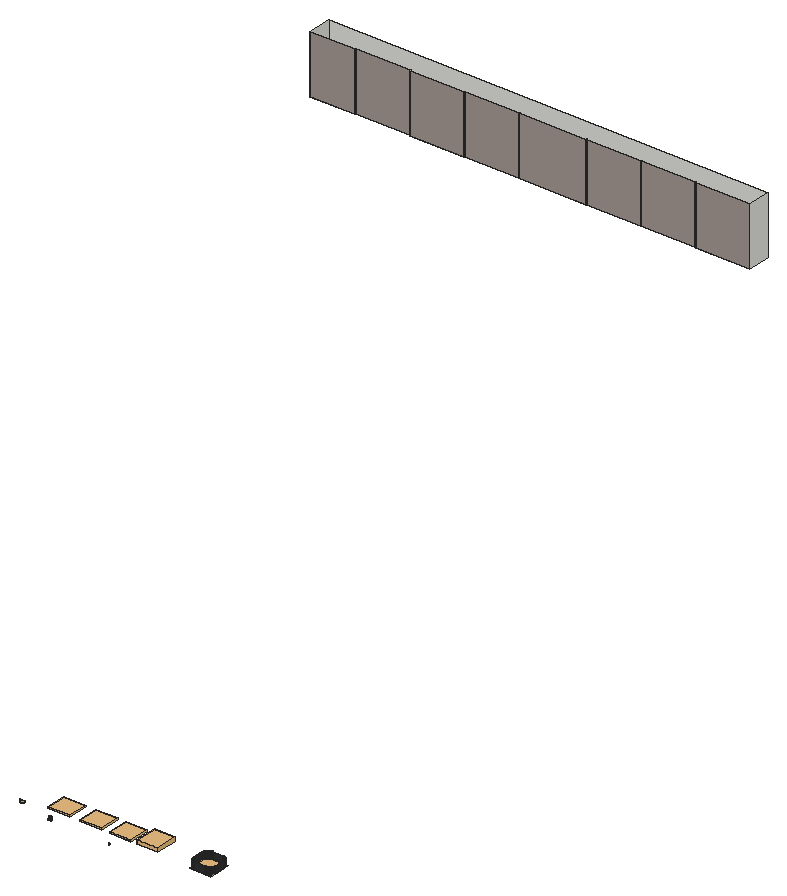
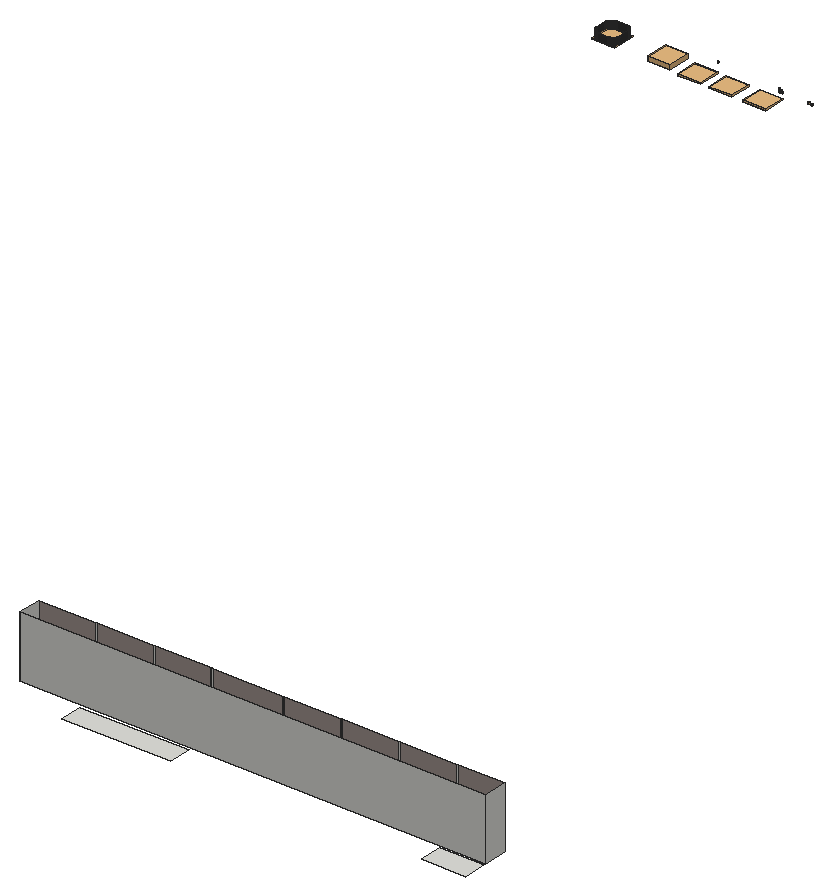
# SketchUp Ruby script. Lengths in inches.
U = 1.inch
M = Sketchup.active_model
def pt(a) = Geom::Point3d.new(a.map { |v| v * U })
def face(e, loops, mat)
  f = e.add_face(loops[0].map { |a| pt(a) })
  loops[1..].each { |l| e.add_face(l.map { |a| pt(a) }).erase! }
  f.material = f.back_material = mat if mat
  f
end
# faces: each face lists its corners as indices into pts; further lists are holes
def faces(e, pts, list, mat = nil) = list.each { |f| face(e, (f[0].is_a?(Array) ? f : [f]).map { |l| l.map { |i| pts[i] } }, mat) }
# xy, xz, yz: faces in a plane at the given z, y or x. An outline is a flat list of corners, or four numbers for a rectangle; further outlines are holes
def ring(l) = l.size == 4 ? [[l[0], l[1]], [l[2], l[1]], [l[2], l[3]], [l[0], l[3]]] : l.each_slice(2).to_a
def flat(e, list, mat, &to3) = list.each { |f| face(e, (f[0].is_a?(Array) ? f : [f]).map { |l| ring(l).map { |u, v| to3.(u, v) } }, mat) }
def xy(e, z, list, mat = nil) = flat(e, list, mat) { |x, y| [x, y, z] }
def xz(e, y, list, mat = nil) = flat(e, list, mat) { |x, z| [x, y, z] }
def yz(e, x, list, mat = nil) = flat(e, list, mat) { |y, z| [x, y, z] }
def lines(e, pts, list) = list.each { |a, b| e.add_line(pt(pts[a]), pt(pts[b])) }
# prism: a flat outline (further loops are holes) pulled along v
def prism(e, loops, v, mat = nil)
  f = face(e, loops, mat); d = Geom::Vector3d.new(v.map { |x| x * U })
  f.pushpull(f.normal.samedirection?(d) ? d.length : -d.length)
end
def box(e, o, s, mat = nil) = prism(e, [[o, [o[0] + s[0], o[1], o[2]], [o[0] + s[0], o[1] + s[1], o[2]], [o[0], o[1] + s[1], o[2]]]], [0, 0, s[2]], mat)
def at(x, y, z, deg = 0) = Geom::Transformation.translation(pt([x, y, z])) * Geom::Transformation.rotation(ORIGIN, Z_AXIS, deg.degrees)
def axes(o, x, y, z) = Geom::Transformation.new([*x, 0, *y, 0, *z, 0, *pt(o).to_a, 1])
def part(name) = M.definitions.add(name)
# library, detail: a bought-in or finely detailed component or shape, given as its bounding box
def library(name, o, s) = part(name).tap { |d| box(d.entities, o, s) }
def detail(e, o, s) = box(e.add_group.entities, o, s)
def put(e, d, t, mat = nil) = e.add_instance(d, t).tap { |i| i.material = mat if mat }
def group(e, t, mat = nil) = e.add_group.tap { |g| g.transformation = t; g.material = mat if mat }.entities
root = M.entities
M.materials.add("11").color = [255, 255, 255]
M.materials.add("21").color = [186, 186, 186]
M.materials.add("23").color = [196, 196, 196]
M.materials.add("25").color = [154, 148, 138]
M.materials.add("8").color = [50, 50, 50]
M.materials.add("[0132_LightGray]").color = [165, 152, 148]
c1 = library("Group91",[37983.22,7255.3125,1514.3125],[8.34,0.24,4.16])
c2 = library("Group92",[38002.24,7255.3125,1514.3125],[8.5,0.24,4.18])
c3 = library("Group90",[37964.07,7255.3125,1514.36],[8.43,0.24,4.13])
c4 = library("om.cn_51698238",[-12277.97,-120000,175247.47],[24687.75,10000,11950.5])
c5 = library("om.cn_53303911",[-146.53,-184.11,-9.51],[291.35,270.38,19.02])
c6 = library("Group18",[-148.91,-148.91,209.88],[297.82,297.82,5])
c7 = library("Group60",[37529.04,7320.21,1549.6],[63.38,1.58,25.46])
c8 = library("Group36",[-8.48,79.83,-140.46],[281.14,53.12,289.99])
xy(root,87.84,[[161.59,558.47,216.39,569.78]])
xy(root,88.02,[[13.72,558.47,35.57,569.78]])
xy(root,88.59,[[[384.77,4.87,384.54,4.875,384.51,4.875,384.47,4.88,384.44,4.88,384.41,4.89,384.34,4.89,384.3125,4.9,384.28,4.9,384.25,4.91,384.22,4.91,384.18,4.92,384.15,4.92,384.12,4.93,384.09,4.9375,383.87,4.99,383.66,5.0625,383.46,5.14,383.26,5.24,383.07,5.35,382.89,5.47,382.72,5.6,382.55,5.74,382.4,5.89,382.26,6.06,382.125,6.23,382.01,6.41,381.9,6.6,381.8,6.8,381.72,7,381.65,7.21,381.6,7.43,381.58,7.49,381.58,7.52,381.57,7.56,381.57,7.59,381.5625,7.62,381.56,7.65,381.55,7.68,381.55,7.75,381.54,7.78,381.54,7.85,381.53,7.88,381.53,13.58,381.54,13.61,381.54,13.68,381.55,13.71,381.55,13.77,381.56,13.81,381.5625,13.84,381.57,13.87,381.57,13.9,381.58,13.93,381.58,13.96,381.59,14,381.6,14.03,381.65,14.24,381.72,14.46,381.8,14.66,381.9,14.86,382.01,15.05,382.125,15.23,382.26,15.4,382.4,15.5625,382.55,15.72,382.72,15.86,382.89,15.99,383.07,16.11,383.26,16.22,383.46,16.3125,383.66,16.4,383.87,16.47,384.09,16.52,384.12,16.53,384.15,16.53,384.18,16.54,384.22,16.54,384.25,16.55,384.28,16.55,384.3125,16.56,384.34,16.5625,384.375,16.57,384.44,16.57,384.47,16.58,384.54,16.58,384.77,16.59,390.01,16.59,390.24,16.58,390.3,16.58,390.34,16.57,390.4,16.57,390.43,16.5625,390.47,16.56,390.5,16.55,390.53,16.55,390.5625,16.54,390.59,16.54,390.625,16.53,390.66,16.53,390.6875,16.52,390.9,16.47,391.12,16.4,391.32,16.3125,391.52,16.22,391.71,16.11,391.89,15.99,392.06,15.86,392.22,15.72,392.375,15.5625,392.52,15.4,392.65,15.23,392.77,15.05,392.88,14.86,393.06,14.46,393.125,14.24,393.18,14.03,393.1875,14,393.19,13.96,393.2,13.93,393.2,13.9,393.21,13.87,393.21,13.84,393.22,13.81,393.22,13.77,393.23,13.74,393.23,13.68,393.24,13.64,393.24,13.58,393.25,13.35,393.25,8.11,393.24,7.88,393.24,7.8125,393.23,7.78,393.23,7.72,393.22,7.68,393.22,7.65,393.21,7.62,393.21,7.59,393.2,7.56,393.2,7.52,393.19,7.49,393.1875,7.46,393.125,7.21,393.06,7,392.88,6.6,392.77,6.41,392.65,6.23,392.52,6.06,392.375,5.89,392.22,5.74,392.06,5.6,391.89,5.47,391.71,5.35,391.52,5.24,391.32,5.14,391.12,5.0625,390.9,4.99,390.6875,4.9375,390.66,4.93,390.625,4.92,390.59,4.92,390.5625,4.91,390.53,4.91,390.5,4.9,390.47,4.9,390.43,4.89,390.37,4.89,390.34,4.88,390.3,4.88,390.27,4.875,390.24,4.875,390.01,4.87],[381.6,13.8,381.64,14.02,381.63,13.99,381.6,13.8,381.625,13.96,381.62,13.93,381.6,13.8,381.61,13.86,381.6,13.83]],[381.6,13.8,381.6,13.83,381.61,13.86],[381.6,13.8,381.62,13.93,381.625,13.96],[381.6,13.8,381.63,13.99,381.64,14.02]],"8")
xy(root,89,[[12.74,546.47,12.74,558.47,246.55,558.47,246.55,546.47,217.85,546.47,217.85,546.77,217.55,546.77,217.55,546.47,188.85,546.47,188.85,546.77,188.55,546.77,188.55,546.47,159.85,546.47,159.85,546.77,159.55,546.77,159.55,546.47,123.85,546.47,123.85,546.77,123.55,546.77,123.55,546.47,94.85,546.47,94.85,546.77,94.55,546.77,94.55,546.47,65.85,546.47,65.85,546.77,65.55,546.77,65.55,546.47,36.85,546.47,36.85,546.77,36.55,546.77,36.55,546.47]])
xz(root,4.87,[[384.77,88.59,390.01,92.32]],"8")
xz(root,4.875,[[384.51,88.59,384.54,92.32],[390.24,88.59,390.27,92.32]],"8")
xz(root,4.88,[[384.44,88.59,384.47,92.32],[390.3,88.59,390.34,92.32]],"8")
xz(root,4.89,[[384.34,88.59,384.375,92.32],[384.375,88.59,384.41,92.32],[390.37,88.59,390.4,92.32],[390.4,88.59,390.43,92.32]],"8")
xz(root,4.9,[[384.28,88.59,384.3125,92.32],[390.47,88.59,390.5,92.32]],"8")
xz(root,4.91,[[384.22,88.59,384.25,92.32],[390.53,88.59,390.5625,92.32]],"8")
xz(root,4.92,[[384.15,88.59,384.18,92.32],[390.59,88.59,390.625,92.32]],"8")
xz(root,16.53,[[384.12,88.59,384.15,92.32],[390.625,88.59,390.66,92.32]],"8")
xz(root,16.54,[[384.18,88.59,384.22,92.32],[390.5625,88.59,390.59,92.32]],"8")
xz(root,16.55,[[384.25,88.59,384.28,92.32],[390.5,88.59,390.53,92.32]],"8")
xz(root,16.57,[[384.375,88.59,384.41,92.32],[384.41,88.59,384.44,92.32],[390.34,88.59,390.37,92.32],[390.37,88.59,390.4,92.32]],"8")
xz(root,16.58,[[384.47,88.59,384.51,92.32],[384.51,88.59,384.54,92.32],[390.24,88.59,390.27,92.32],[390.27,88.59,390.3,92.32]],"8")
xz(root,16.59,[[384.77,88.59,390.01,92.32]],"8")
xz(root,546.47,[[12.74,89,36.55,120],[36.85,89,65.55,120],[65.85,89,94.55,120],[94.85,89,123.55,120],[123.85,89,159.55,120],
  [159.85,89,188.55,120],[188.85,89,217.55,120],[217.85,89,246.55,120]],"[0132_LightGray]")
xz(root,546.77,[[36.55,89,36.85,120],[65.55,89,65.85,120],[94.55,89,94.85,120],[123.55,89,123.85,120],[159.55,89,159.85,120],
  [188.55,89,188.85,120],[217.55,89,217.85,120]])
xz(root,558.47,[[12.74,89,246.55,120]])
yz(root,12.74,[[546.47,89,558.47,120]])
yz(root,36.55,[[546.47,89,546.77,120]])
yz(root,36.85,[[546.47,89,546.77,120]])
yz(root,65.55,[[546.47,89,546.77,120]])
yz(root,65.85,[[546.47,89,546.77,120]])
yz(root,94.55,[[546.47,89,546.77,120]])
yz(root,94.85,[[546.47,89,546.77,120]])
yz(root,123.55,[[546.47,89,546.77,120]])
yz(root,123.85,[[546.47,89,546.77,120]])
yz(root,159.55,[[546.47,89,546.77,120]])
yz(root,159.85,[[546.47,89,546.77,120]])
yz(root,188.55,[[546.47,89,546.77,120]])
yz(root,188.85,[[546.47,89,546.77,120]])
yz(root,217.55,[[546.47,89,546.77,120]])
yz(root,217.85,[[546.47,89,546.77,120]])
yz(root,246.55,[[546.47,89,558.47,120]])
yz(root,381.53,[[7.88,88.59,8.11,92.32],[8.11,88.59,13.35,92.32],[13.35,88.59,13.58,92.32]],"8")
yz(root,381.54,[[7.78,88.59,7.8125,92.32],[7.8125,88.59,7.85,92.32],[13.61,88.59,13.64,92.32],[13.64,88.59,13.68,92.32]],"8")
yz(root,381.55,[[7.68,88.59,7.72,92.32],[7.72,88.59,7.75,92.32],[13.71,88.59,13.74,92.32],[13.74,88.59,13.77,92.32]],"8")
yz(root,381.57,[[7.56,88.59,7.59,92.32],[13.87,88.59,13.9,92.32]],"8")
yz(root,381.58,[[7.49,88.59,7.52,92.32],[13.93,88.59,13.96,92.32]],"8")
yz(root,393.2,[[7.52,88.59,7.56,92.32],[13.9,88.59,13.93,92.32]],"8")
yz(root,393.21,[[7.59,88.59,7.62,92.32],[13.84,88.59,13.87,92.32]],"8")
yz(root,393.22,[[7.65,88.59,7.68,92.32],[13.77,88.59,13.81,92.32]],"8")
yz(root,393.23,[[7.72,88.59,7.75,92.32],[7.75,88.59,7.78,92.32],[13.68,88.59,13.71,92.32],[13.71,88.59,13.74,92.32]],"8")
yz(root,393.24,[[7.8125,88.59,7.85,92.32],[7.85,88.59,7.88,92.32],[13.58,88.59,13.61,92.32],[13.61,88.59,13.64,92.32]],"8")
yz(root,393.25,[[8.11,88.59,13.35,92.32]],"8")
p = [[383.87,4.99,92.32],[383.87,4.99,88.59],[384.09,4.9375,88.59],[384.09,4.9375,92.32],[384.12,4.93,88.59],[384.12,4.93,92.32],
  [384.15,4.92,88.59],[384.15,4.92,92.32],[384.25,4.91,92.32],[384.25,4.91,88.59],[384.28,4.9,88.59],[384.28,4.9,92.32],
  [384.18,4.92,92.32],[384.18,4.92,88.59],[384.22,4.91,88.59],[384.22,4.91,92.32],[384.3125,4.9,92.32],[384.3125,4.9,88.59],
  [384.34,4.89,88.59],[384.34,4.89,92.32],[384.41,4.89,92.32],[384.41,4.89,88.59],[384.44,4.88,88.59],[384.44,4.88,92.32],
  [384.47,4.88,92.32],[384.47,4.88,88.59],[384.51,4.875,88.59],[384.51,4.875,92.32],[384.54,4.875,92.32],[384.54,4.875,88.59],
  [384.77,4.87,88.59],[384.77,4.87,92.32],[390.01,4.87,92.32],[390.01,4.87,88.59],[390.24,4.875,88.59],[390.24,4.875,92.32],
  [390.34,4.88,92.32],[390.34,4.88,88.59],[390.37,4.89,88.59],[390.37,4.89,92.32],[390.27,4.875,92.32],[390.27,4.875,88.59],
  [390.3,4.88,88.59],[390.3,4.88,92.32],[390.43,4.89,92.32],[390.43,4.89,88.59],[390.47,4.9,88.59],[390.47,4.9,92.32],
  [390.5,4.9,92.32],[390.5,4.9,88.59],[390.53,4.91,88.59],[390.53,4.91,92.32],[390.625,4.92,92.32],[390.625,4.92,88.59],
  [390.66,4.93,88.59],[390.66,4.93,92.32],[390.5625,4.91,92.32],[390.5625,4.91,88.59],[390.59,4.92,88.59],[390.59,4.92,92.32],
  [390.6875,4.9375,88.59],[390.6875,4.9375,92.32],[390.9,4.99,88.59],[390.9,4.99,92.32],[383.66,5.0625,92.32],[383.66,5.0625,88.59],
  [391.12,5.0625,88.59],[391.12,5.0625,92.32],[383.26,5.24,92.32],[383.26,5.24,88.59],[383.46,5.14,88.59],[383.46,5.14,92.32],
  [391.32,5.14,88.59],[391.32,5.14,92.32],[391.52,5.24,88.59],[391.52,5.24,92.32],[383.07,5.35,92.32],[383.07,5.35,88.59],
  [391.71,5.35,88.59],[391.71,5.35,92.32],[382.89,5.47,92.32],[382.89,5.47,88.59],[391.89,5.47,88.59],[391.89,5.47,92.32],
  [382.72,5.6,92.32],[382.72,5.6,88.59],[392.06,5.6,88.59],[392.06,5.6,92.32],[382.55,5.74,92.32],[382.55,5.74,88.59],
  [392.22,5.74,88.59],[392.22,5.74,92.32],[382.4,5.89,92.32],[382.4,5.89,88.59],[392.375,5.89,88.59],[392.375,5.89,92.32],
  [382.26,6.06,92.32],[382.26,6.06,88.59],[392.52,6.06,88.59],[392.52,6.06,92.32],[382.125,6.23,92.32],[382.125,6.23,88.59],
  [392.65,6.23,88.59],[392.65,6.23,92.32],[382.01,6.41,92.32],[382.01,6.41,88.59],[392.77,6.41,88.59],[392.77,6.41,92.32],
  [381.9,6.6,92.32],[381.9,6.6,88.59],[392.88,6.6,88.59],[392.88,6.6,92.32],[381.8,6.8,92.32],[381.8,6.8,88.59],
  [392.97,6.8,88.59],[392.97,6.8,92.32],[381.72,7,92.32],[381.72,7,88.59],[393.06,7,88.59],[393.06,7,92.32],
  [381.65,7.21,92.32],[381.65,7.21,88.59],[393.125,7.21,88.59],[393.125,7.21,92.32],[381.6,7.43,92.32],[381.6,7.43,88.59],
  [393.18,7.43,88.59],[393.18,7.43,92.32],[381.59,7.46,92.32],[381.59,7.46,88.59],[393.1875,7.46,88.59],[393.1875,7.46,92.32],
  [381.58,7.49,92.32],[381.58,7.49,88.59],[381.57,7.56,92.32],[381.57,7.56,88.59],[381.58,7.52,88.59],[381.58,7.52,92.32],
  [393.19,7.49,88.59],[393.19,7.49,92.32],[393.2,7.52,88.59],[393.2,7.52,92.32],[381.5625,7.62,92.32],[381.5625,7.62,88.59],
  [381.57,7.59,88.59],[381.57,7.59,92.32],[381.56,7.65,92.32],[381.56,7.65,88.59],[393.2,7.56,92.32],[393.2,7.56,88.59],
  [393.21,7.59,88.59],[393.21,7.59,92.32],[393.21,7.62,92.32],[393.21,7.62,88.59],[393.22,7.65,88.59],[393.22,7.65,92.32],
  [381.54,7.78,92.32],[381.54,7.78,88.59],[381.55,7.75,88.59],[381.55,7.75,92.32],[381.55,7.68,92.32],[381.55,7.68,88.59],
  [393.22,7.68,92.32],[393.22,7.68,88.59],[393.23,7.72,88.59],[393.23,7.72,92.32],[381.53,7.88,92.32],[381.53,7.88,88.59],
  [381.54,7.85,88.59],[381.54,7.85,92.32],[393.23,7.78,92.32],[393.23,7.78,88.59],[393.24,7.8125,88.59],[393.24,7.8125,92.32],
  [393.24,7.88,92.32],[393.24,7.88,88.59],[393.25,8.11,88.59],[393.25,8.11,92.32],[393.25,13.35,92.32],[393.25,13.35,88.59],
  [393.24,13.58,88.59],[393.24,13.58,92.32],[381.54,13.61,92.32],[381.54,13.61,88.59],[381.53,13.58,88.59],[381.53,13.58,92.32],
  [393.24,13.64,92.32],[393.24,13.64,88.59],[393.23,13.68,88.59],[393.23,13.68,92.32],[381.55,13.71,92.32],[381.55,13.71,88.59],
  [381.54,13.68,88.59],[381.54,13.68,92.32],[393.23,13.74,92.32],[393.23,13.74,88.59],[393.22,13.77,88.59],[393.22,13.77,92.32],
  [381.5625,13.84,92.32],[381.5625,13.84,88.59],[381.56,13.81,88.59],[381.56,13.81,92.32],[381.55,13.77,88.59],[381.55,13.77,92.32],
  [381.57,13.87,92.32],[381.57,13.87,88.59],[393.22,13.81,92.32],[393.22,13.81,88.59],[393.21,13.84,88.59],[393.21,13.84,92.32],
  [381.58,13.93,92.32],[381.58,13.93,88.59],[381.57,13.9,88.59],[381.57,13.9,92.32],[393.21,13.87,92.32],[393.21,13.87,88.59],
  [393.2,13.9,88.59],[393.2,13.9,92.32],[393.2,13.93,92.32],[393.2,13.93,88.59],[393.19,13.96,88.59],[393.19,13.96,92.32],
  [381.65,14.24,92.32],[381.65,14.24,88.59],[381.6,14.03,88.59],[381.6,14.03,92.32],[381.59,14,88.59],[381.59,14,92.32],
  [381.58,13.96,88.59],[381.58,13.96,92.32],[393.18,14.03,92.32],[393.18,14.03,88.59],[393.125,14.24,88.59],[393.125,14.24,92.32],
  [393.1875,14,88.59],[393.1875,14,92.32],[381.72,14.46,92.32],[381.72,14.46,88.59],[393.06,14.46,88.59],[393.06,14.46,92.32],
  [381.8,14.66,92.32],[381.8,14.66,88.59],[392.97,14.66,88.59],[392.97,14.66,92.32],[381.9,14.86,92.32],[381.9,14.86,88.59],
  [392.88,14.86,88.59],[392.88,14.86,92.32],[382.01,15.05,92.32],[382.01,15.05,88.59],[392.77,15.05,88.59],[392.77,15.05,92.32],
  [382.125,15.23,92.32],[382.125,15.23,88.59],[392.65,15.23,88.59],[392.65,15.23,92.32],[382.26,15.4,92.32],[382.26,15.4,88.59],
  [392.52,15.4,88.59],[392.52,15.4,92.32],[382.4,15.5625,92.32],[382.4,15.5625,88.59],[392.375,15.5625,88.59],[392.375,15.5625,92.32],
  [382.55,15.72,92.32],[382.55,15.72,88.59],[392.22,15.72,88.59],[392.22,15.72,92.32],[382.72,15.86,92.32],[382.72,15.86,88.59],
  [392.06,15.86,88.59],[392.06,15.86,92.32],[382.89,15.99,92.32],[382.89,15.99,88.59],[391.89,15.99,88.59],[391.89,15.99,92.32],
  [383.07,16.11,92.32],[383.07,16.11,88.59],[391.71,16.11,88.59],[391.71,16.11,92.32],[383.26,16.22,92.32],[383.26,16.22,88.59],
  [391.52,16.22,88.59],[391.52,16.22,92.32],[383.46,16.3125,92.32],[383.46,16.3125,88.59],[391.32,16.3125,88.59],[391.32,16.3125,92.32],
  [383.66,16.4,92.32],[383.66,16.4,88.59],[391.12,16.4,88.59],[391.12,16.4,92.32],[383.87,16.47,92.32],[383.87,16.47,88.59],
  [390.9,16.47,88.59],[390.9,16.47,92.32],[384.09,16.52,92.32],[384.09,16.52,88.59],[384.12,16.53,92.32],[384.12,16.53,88.59],
  [384.18,16.54,92.32],[384.18,16.54,88.59],[384.15,16.53,88.59],[384.15,16.53,92.32],[384.25,16.55,92.32],[384.25,16.55,88.59],
  [384.22,16.54,88.59],[384.22,16.54,92.32],[390.5625,16.54,92.32],[390.5625,16.54,88.59],[390.53,16.55,88.59],[390.53,16.55,92.32],
  [390.625,16.53,92.32],[390.625,16.53,88.59],[390.59,16.54,88.59],[390.59,16.54,92.32],[390.6875,16.52,88.59],[390.6875,16.52,92.32],
  [390.66,16.53,88.59],[390.66,16.53,92.32],[384.375,16.57,92.32],[384.375,16.57,88.59],[384.34,16.5625,88.59],[384.34,16.5625,92.32],
  [384.3125,16.56,88.59],[384.3125,16.56,92.32],[384.28,16.55,88.59],[384.28,16.55,92.32],[384.47,16.58,92.32],[384.47,16.58,88.59],
  [384.44,16.57,88.59],[384.44,16.57,92.32],[384.77,16.59,92.32],[384.77,16.59,88.59],[384.54,16.58,88.59],[384.54,16.58,92.32],
  [390.24,16.58,92.32],[390.24,16.58,88.59],[390.01,16.59,88.59],[390.01,16.59,92.32],[390.34,16.57,92.32],[390.34,16.57,88.59],
  [390.3,16.58,88.59],[390.3,16.58,92.32],[390.47,16.56,92.32],[390.47,16.56,88.59],[390.43,16.5625,88.59],[390.43,16.5625,92.32],
  [390.4,16.57,88.59],[390.4,16.57,92.32],[390.5,16.55,92.32],[390.5,16.55,88.59]]
faces(root,p,[[0,1,2,3],[3,2,4,5],[5,4,6,7],[8,9,10,11],[12,13,14,15],[16,17,18,19],[20,21,22,23],[24,25,26,27],
  [28,29,30,31],[32,33,34,35],[36,37,38,39],[40,41,42,43],[44,45,46,47],[48,49,50,51],[52,53,54,55],[56,57,58,59],
  [55,54,60,61],[61,60,62,63],[64,65,1,0],[63,62,66,67],[68,69,70,71],[71,70,65,64],[67,66,72,73],[73,72,74,75],
  [76,77,69,68],[75,74,78,79],[80,81,77,76],[79,78,82,83],[84,85,81,80],[83,82,86,87],[88,89,85,84],[87,86,90,91],
  [92,93,89,88],[91,90,94,95],[96,97,93,92],[95,94,98,99],[100,101,97,96],[99,98,102,103],[104,105,101,100],[103,102,106,107],
  [108,109,105,104],[107,106,110,111],[112,113,109,108],[111,110,114,115],[116,117,113,112],[115,114,118,119],[120,121,117,116],[119,118,122,123],
  [124,125,121,120],[123,122,126,127],[128,129,125,124],[127,126,130,131],[132,133,129,128],[134,135,136,137],[131,130,138,139],[139,138,140,141],
  [142,143,144,145],[146,147,143,142],[148,149,150,151],[152,153,154,155],[156,157,158,159],[160,161,147,146],[162,163,164,165],[166,167,168,169],
  [170,171,172,173],[174,175,176,177],[178,179,180,181],[182,183,184,185],[186,187,188,189],[190,191,192,193],[194,195,196,197],[198,199,200,201],
  [201,200,202,203],[204,205,199,198],[206,207,208,209],[210,211,212,213],[214,215,216,217],[218,219,220,221],[222,223,224,225],[225,224,226,227],
  [227,226,228,229],[230,231,232,233],[221,220,234,235],[235,234,231,230],[236,237,223,222],[233,232,238,239],[240,241,237,236],[239,238,242,243],
  [244,245,241,240],[243,242,246,247],[248,249,245,244],[247,246,250,251],[252,253,249,248],[251,250,254,255],[256,257,253,252],[255,254,258,259],
  [260,261,257,256],[259,258,262,263],[264,265,261,260],[263,262,266,267],[268,269,265,264],[267,266,270,271],[272,273,269,268],[271,270,274,275],
  [276,277,273,272],[275,274,278,279],[280,281,277,276],[279,278,282,283],[284,285,281,280],[283,282,286,287],[288,289,285,284],[287,286,290,291],
  [292,293,289,288],[291,290,294,295],[296,297,293,292],[298,299,297,296],[300,301,302,303],[304,305,306,307],[308,309,310,311],[312,313,314,315],
  [295,294,316,317],[317,316,318,319],[320,321,322,323],[323,322,324,325],[325,324,326,327],[328,329,330,331],[332,333,334,335],[336,337,338,339],
  [340,341,342,343],[344,345,346,347],[347,346,348,349],[350,351,345,344]],"8")
g1 = group(root,at(-1185.85,-283.55,27.72))
detail(g1,[1495.26,285.64,59.41],[0.59,0.01,0.59])
g2 = group(root,at(-1185.85,-283.55,27.72))
detail(g2,[1494.51,285.64,59.41],[0.59,0.01,0.59])
g3 = group(root,at(-1185.85,-283.55,27.72))
detail(g3,[1496.01,285.64,59.41],[0.59,0.01,0.59])
put(root,c1,axes([-1185.85,-283.55,27.72],[0.03937,0,0],[0,0.03937,0],[0,0,0.03937]))
put(root,c2,axes([-1185.85,-283.55,27.72],[0.03937,0,0],[0,0.03937,0],[0,0,0.03937]))
put(root,c3,axes([-1185.85,-283.55,27.72],[0.03937,0,0],[0,0.03937,0],[0,0,0.03937]))
put(root,c4,axes([309.68,1.17,77.77],[0.00006,0,0],[0,-0.00001,0],[0,0,0.00006]),"11")
g4 = group(root,at(342.9,0.95,86.8))
prism(g4,[[[0.155,-0.945,1.805],[0,-0.945,1.727],[-0.154,-0.945,1.805],[-0.154,-0.945,1.69],[-0.232,-0.945,1.721],[-0.232,-0.945,1.902],[-0.167,-0.945,1.902],[0,-0.945,1.805],[0.168,-0.945,1.902],[0.232,-0.945,1.902],[0.232,-0.945,1.533],[0.154,-0.945,1.565],[0.155,-0.945,1.567],[0.155,-0.945,1.57]]],[0,0.041,0],"11")
detail(g4,[-0.23,-0.95,1.3],[0.45,0.05,0.34])
put(root,c5,axes([342.91,14.81,88.75],[0.03937,0,0],[0,0.03937,0],[0,0,0.03937]),"21")
put(root,c5,axes([326.9,14.99,88.75],[0.03937,0,0],[0,0.03937,0],[0,0,0.03937]),"23")
put(root,c5,axes([309.76,15.12,88.75],[0.03937,0,0],[0,0.03937,0],[0,0,0.03937]),"25")
put(root,c6,axes([387.39,10.73,80.1875],[0.03799,0,0],[0,0.03799,0],[0,0,0.03937]))
put(root,c7,axes([-1185.85,-283.55,27.72],[0.03937,0,0],[0,0.03937,0],[0,0,0.03937]))
put(root,c8,axes([353.2,12.12,86.11],[0.03937,0,0],[0,0,0.03937],[0,-0.03937,0]))
